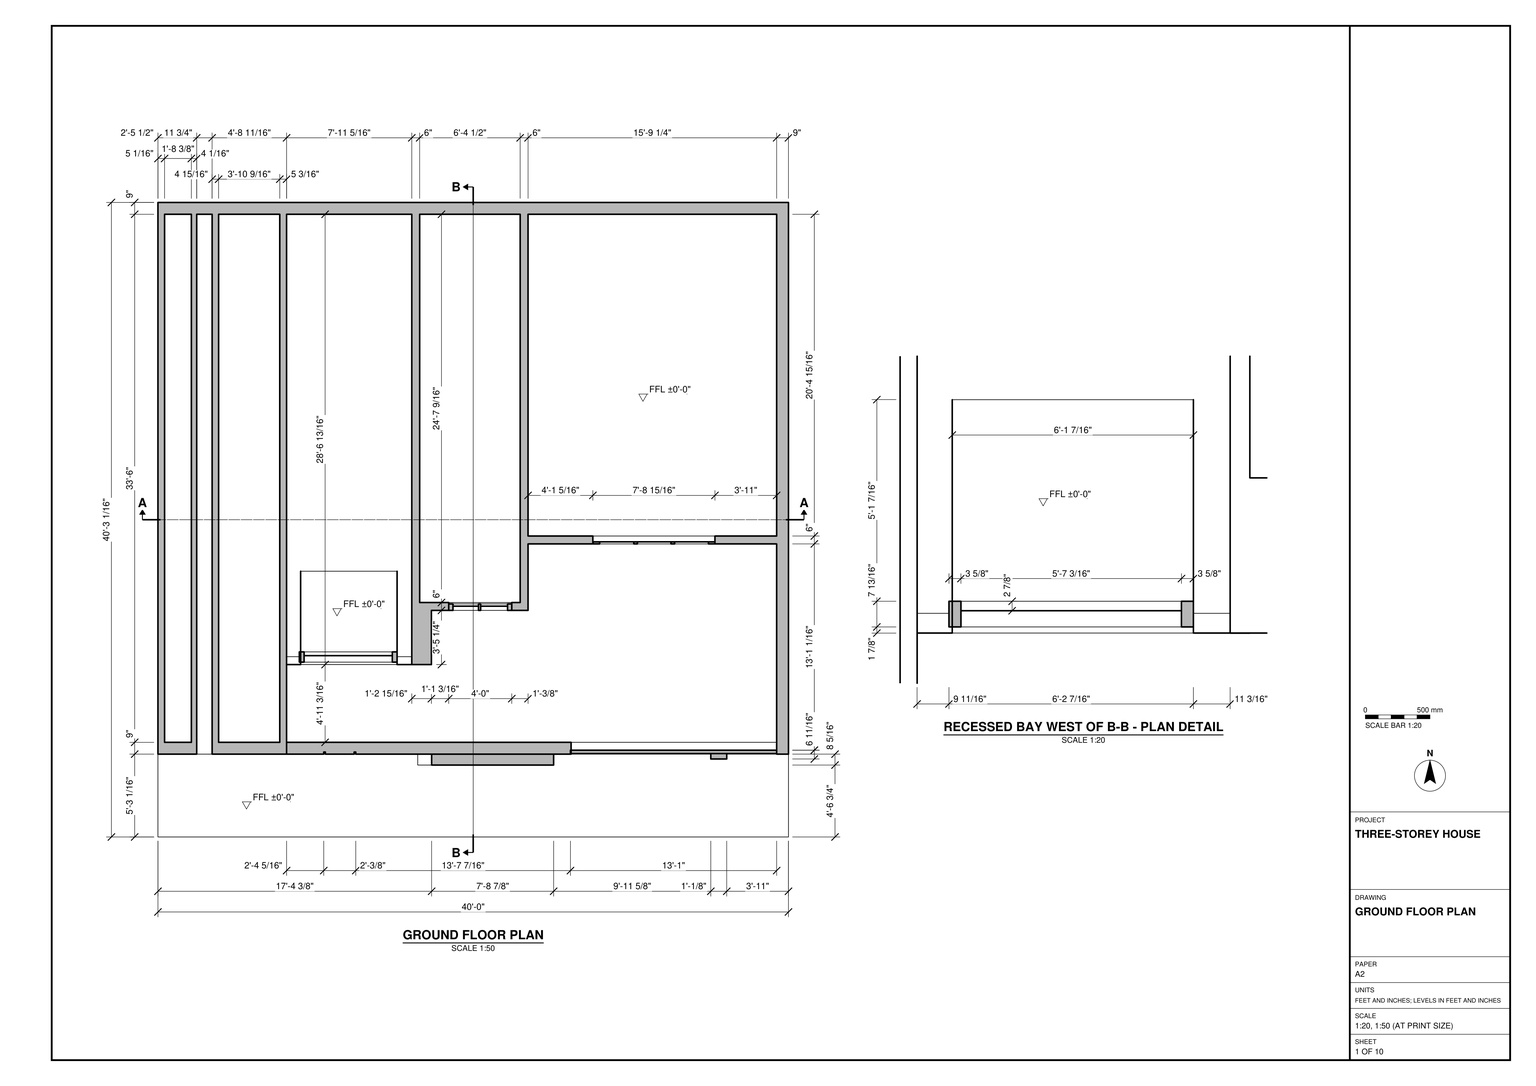
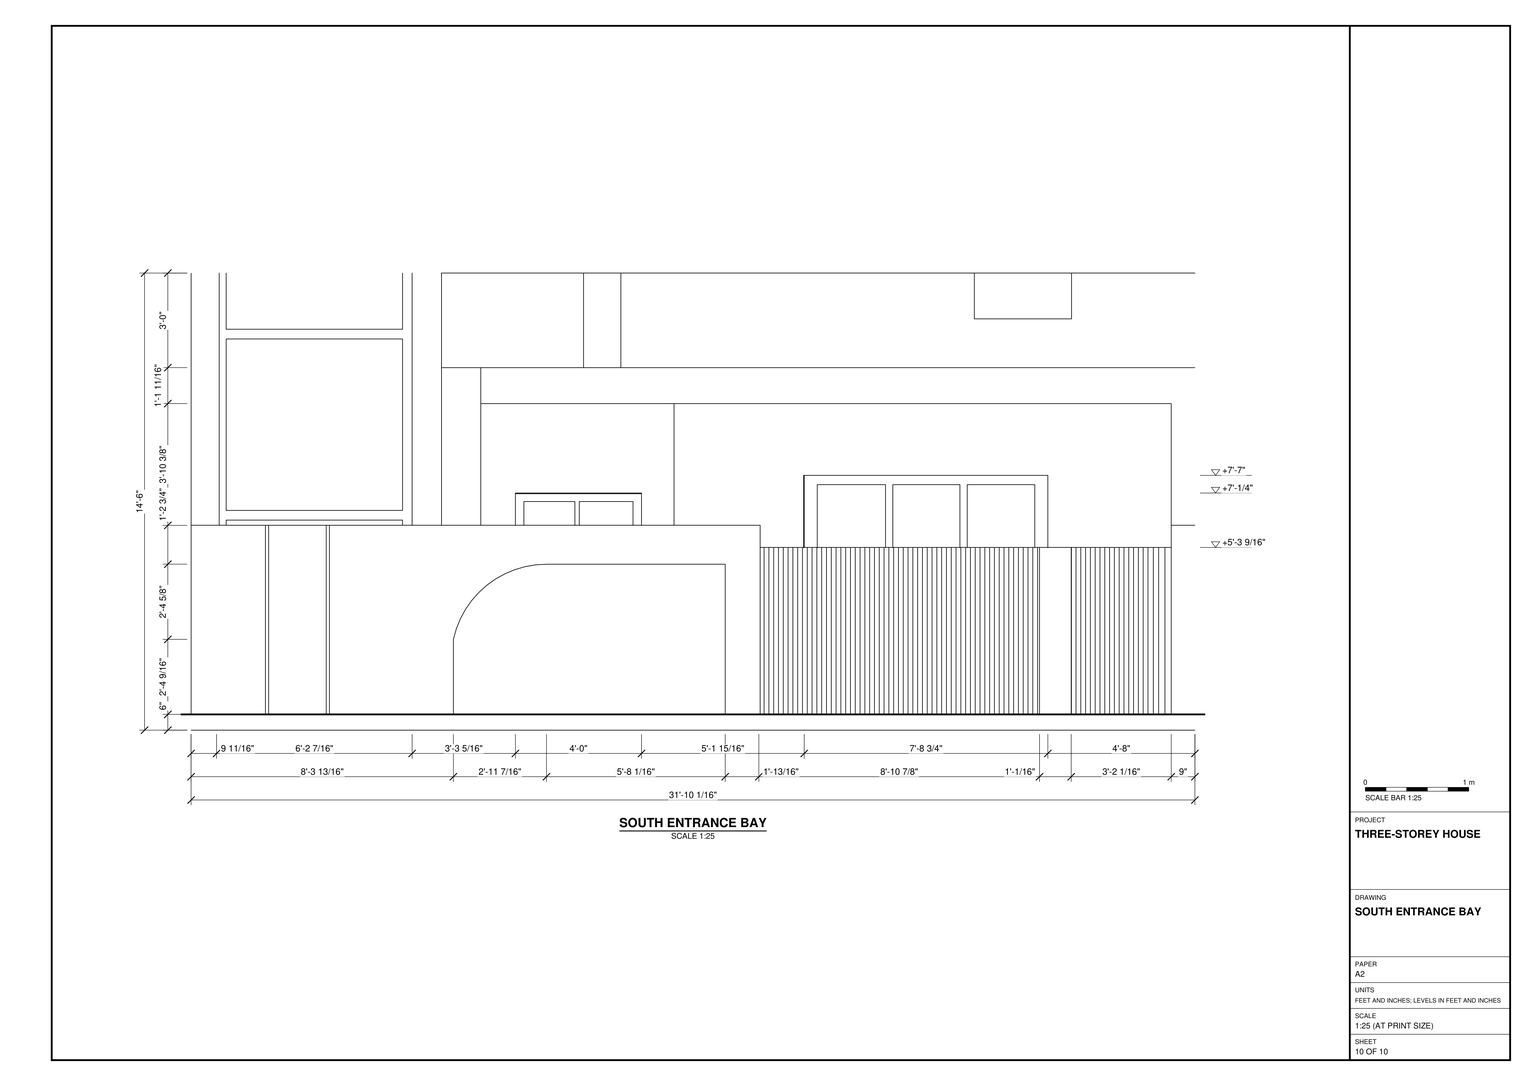
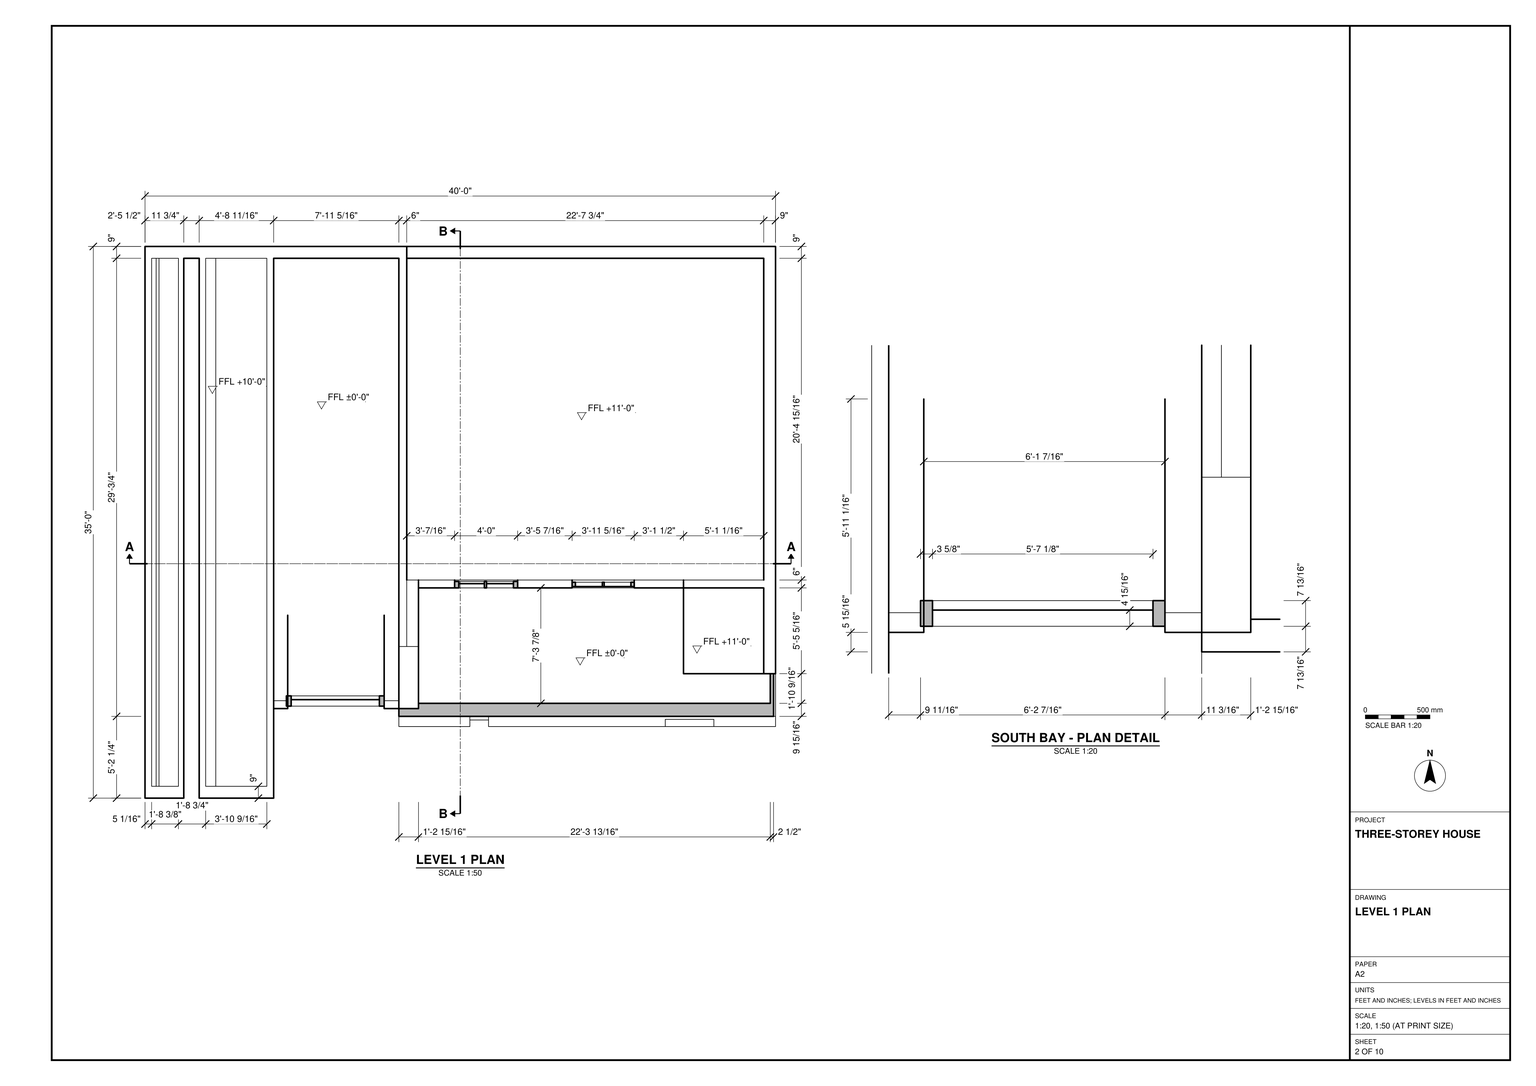
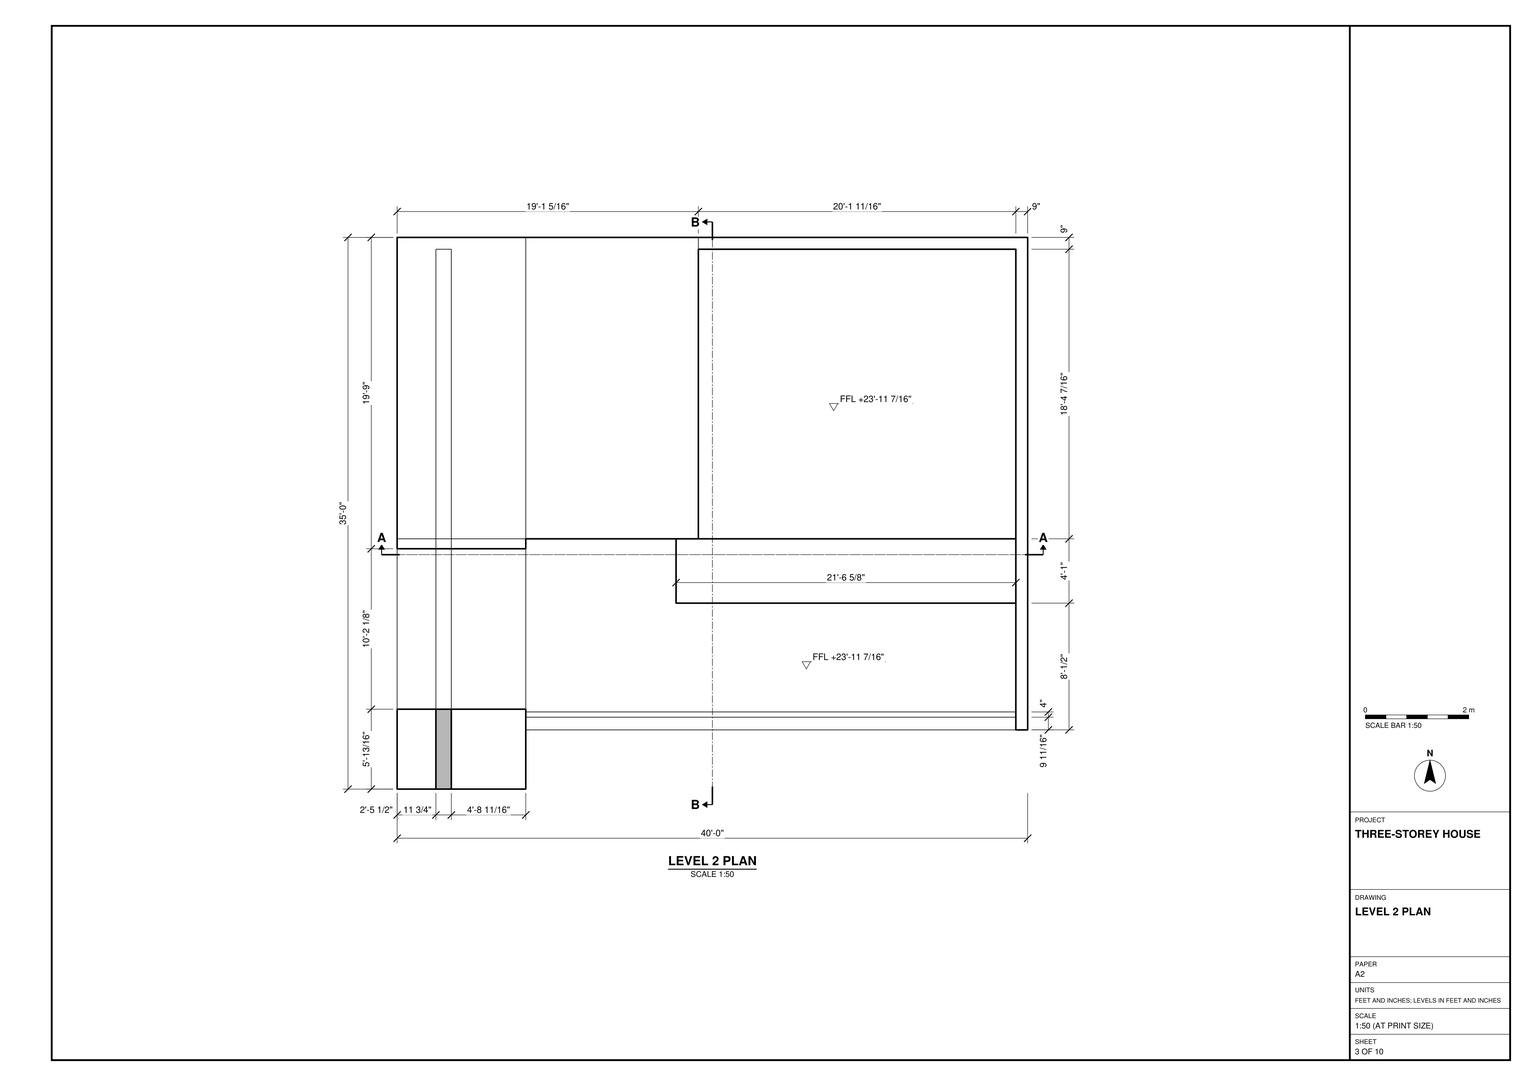
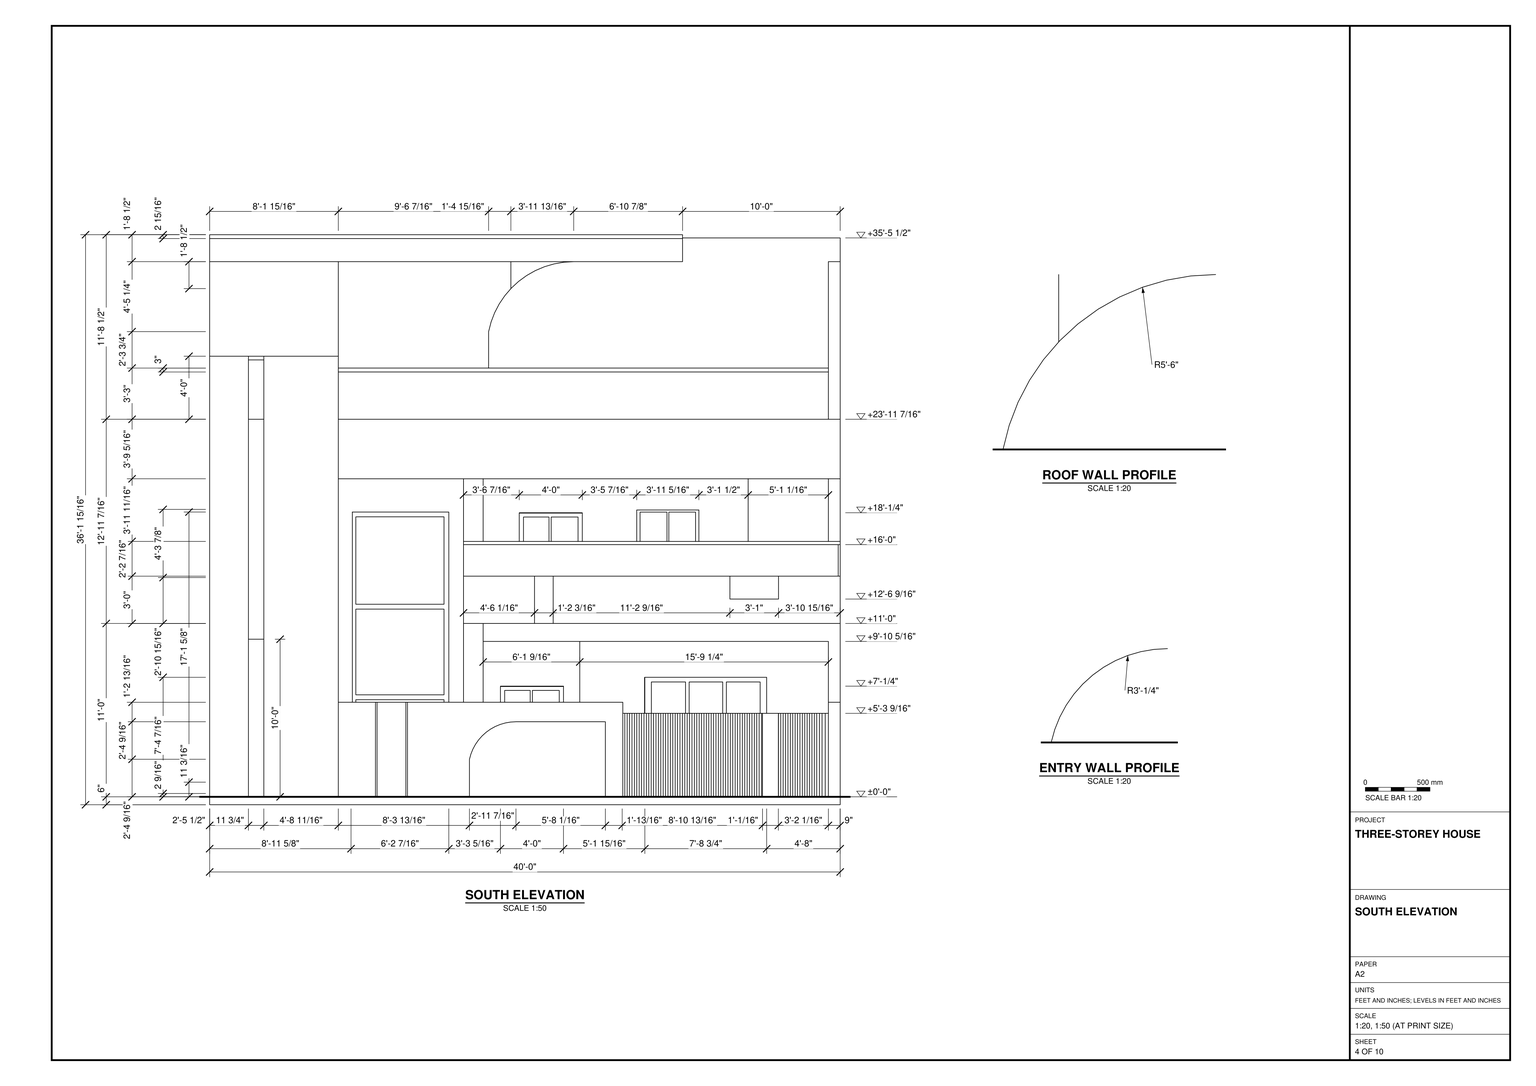
Build the three-storey house in SketchUp using task_files/diagram_01.pdf. Work in feet and inches. The overall model measures 40'-0" east to west, 40'-3 1/16" north to south and 36'-1 15/16" high. Set the finished floor levels at ±0'-0", +11'-0" and +23'-11 7/16".

Use the plans to lay out the long, narrow bays on the west and the wider spaces on the east. Give walls their drawn thicknesses, including 9" and 6" where marked. Form the recessed south bay with its opening set between the side returns. Use each storey's own slab outline rather than copying the ground floor upwards. Preserve the areas open to the floor below, and follow the sheets for the upper walls, openings, stairs and roof.

Use the enlarged south entrance drawing to position the framed openings behind the entrance screen. Match the curved corner profile in the solid portion and the two runs of closely spaced vertical members to its right. Include built-in joinery and main furniture where shown. Keep walls, slabs, roof elements and each furniture or joinery piece in separate groups or components, and use components for repeated parts. Any decor or loose items shown may use suitable library components. Save one SketchUp model as output_files/three_storey_house_with_a_screened_south_entrance.skp.

# SketchUp Ruby script. Lengths in inches.
U = 1.inch
M = Sketchup.active_model
def pt(a) = Geom::Point3d.new(a.map { |v| v * U })
def face(e, loops, mat)
  f = e.add_face(loops[0].map { |a| pt(a) })
  loops[1..].each { |l| e.add_face(l.map { |a| pt(a) }).erase! }
  f.material = f.back_material = mat if mat
  f
end
# faces: each face lists its corners as indices into pts; further lists are holes
def faces(e, pts, list, mat = nil) = list.each { |f| face(e, (f[0].is_a?(Array) ? f : [f]).map { |l| l.map { |i| pts[i] } }, mat) }
# xy, xz, yz: faces in a plane at the given z, y or x. An outline is a flat list of corners, or four numbers for a rectangle; further outlines are holes
def ring(l) = l.size == 4 ? [[l[0], l[1]], [l[2], l[1]], [l[2], l[3]], [l[0], l[3]]] : l.each_slice(2).to_a
def flat(e, list, mat, &to3) = list.each { |f| face(e, (f[0].is_a?(Array) ? f : [f]).map { |l| ring(l).map { |u, v| to3.(u, v) } }, mat) }
def xy(e, z, list, mat = nil) = flat(e, list, mat) { |x, y| [x, y, z] }
def xz(e, y, list, mat = nil) = flat(e, list, mat) { |x, z| [x, y, z] }
def yz(e, x, list, mat = nil) = flat(e, list, mat) { |y, z| [x, y, z] }
def lines(e, pts, list) = list.each { |a, b| e.add_line(pt(pts[a]), pt(pts[b])) }
# prism: a flat outline (further loops are holes) pulled along v
def prism(e, loops, v, mat = nil)
  f = face(e, loops, mat); d = Geom::Vector3d.new(v.map { |x| x * U })
  f.pushpull(f.normal.samedirection?(d) ? d.length : -d.length)
end
def box(e, o, s, mat = nil) = prism(e, [[o, [o[0] + s[0], o[1], o[2]], [o[0] + s[0], o[1] + s[1], o[2]], [o[0], o[1] + s[1], o[2]]]], [0, 0, s[2]], mat)
def at(x, y, z, deg = 0) = Geom::Transformation.translation(pt([x, y, z])) * Geom::Transformation.rotation(ORIGIN, Z_AXIS, deg.degrees)
def axes(o, x, y, z) = Geom::Transformation.new([*x, 0, *y, 0, *z, 0, *pt(o).to_a, 1])
def part(name) = M.definitions.add(name)
# library, detail: a bought-in or finely detailed component or shape, given as its bounding box
def library(name, o, s) = part(name).tap { |d| box(d.entities, o, s) }
def detail(e, o, s) = box(e.add_group.entities, o, s)
def put(e, d, t, mat = nil) = e.add_instance(d, t).tap { |i| i.material = mat if mat }
def group(e, t, mat = nil) = e.add_group.tap { |g| g.transformation = t; g.material = mat if mat }.entities
root = M.entities
M.materials.add("[Color B04]").color = [229, 179, 115]
M.materials.add("[Color B08]").color = [73, 25, 0]
M.materials.add("[Color C02]").color = [255, 204, 153]
M.materials.add("[Color C07]").color = [102, 54, 0]
M.materials.add("[Color M00]").color = [255, 255, 255]
M.materials.add("[Color M05]").color = [114, 114, 114]
M.materials.add("[Concrete Aggregate Smoke]").color = [154, 150, 148]
M.materials.add("[Concrete Form 4x8]").color = [167, 170, 168]
M.materials.add("[Field Rectangle Tile]").color = [196, 189, 179]
M.materials.add("[Field Square Tile]").color = [217, 201, 169]
M.materials.add("[Marble Carrara Gold Floor Tile]").color = [225, 223, 217]
M.materials.add("[Marble Carrara Gold Floor Tile]1").color = [225, 223, 217]
M.materials.add("[Sandstone]").color = [118, 81, 52]
M.materials.add("[Stone Brushed Khaki]").color = [226, 197, 133]
M.materials.add("[Stone Marble]").color = [143, 138, 136]
M.materials.add("[Translucent Glass Blue]").color = [223, 205, 74]
M.materials["[Translucent Glass Blue]"].alpha = 0.5
M.materials.add("[Translucent Glass Gray]").color = [128, 128, 128]
M.materials["[Translucent Glass Gray]"].alpha = 0.5
c1 = part("Group\#3")
xy(c1.entities,0,[[0,0,48,6.5]],"[Color C07]")
xy(c1.entities,3.23,[[22.64,0,24.3125,6.5]])
xy(c1.entities,3.23,[[3.23,0,22.64,4.25],[24.3125,0,44.77,4.25],[3.23,4.25,22.64,6.5],[24.3125,4.25,44.77,6.5]],"[Color C07]")
xy(c1.entities,80.77,[[3.23,0,22.64,4.25],[24.3125,0,44.77,4.25],[3.23,4.25,22.64,6.5],[24.3125,4.25,44.77,6.5]],"[Color C07]")
xy(c1.entities,84,[[0,0,48,6.5]],"[Color C07]")
xz(c1.entities,0,[[[0,0,48,84],[3.23,3.23,3.23,80.77,22.64,80.77,22.64,3.23,24.3125,3.23,24.3125,80.77,44.77,80.77,44.77,3.23]]],"[Color C07]")
xz(c1.entities,4.25,[[3.23,3.23,22.64,80.77],[24.3125,3.23,44.77,80.77]],"[Color C07]")
xz(c1.entities,6.5,[[[0,0,48,84],[3.23,3.23,44.77,3.23,44.77,80.77,24.3125,80.77,24.3125,3.23,22.64,3.23,22.64,80.77,3.23,80.77]]],"[Color C07]")
yz(c1.entities,0,[[0,0,6.5,84]],"[Color C07]")
yz(c1.entities,3.23,[[0,3.23,4.25,80.77],[4.25,3.23,6.5,80.77]],"[Color C07]")
yz(c1.entities,22.64,[[0,3.23,4.25,80.77],[4.25,3.23,6.5,80.77]],"[Color C07]")
yz(c1.entities,24.3125,[[0,3.23,4.25,80.77],[4.25,3.23,6.5,80.77]],"[Color C07]")
yz(c1.entities,44.77,[[0,3.23,4.25,80.77],[4.25,3.23,6.5,80.77]],"[Color C07]")
yz(c1.entities,48,[[0,0,6.5,84]],"[Color C07]")
xy(root,0,[[0,0,480,63.0625],[0,63.0625,480,483.0625]],"[Concrete Form 4x8]")
xy(root,6,[[[0,63.0625,0,483.0625,45.375,483.0625,45.375,474.0625,29.52,474.0625,29.52,63.0625],[5.0625,72.0625,25.4375,474.0625]],[29.52,63.0625,41.25,474.0625],[41.25,63.0625,41.25,474.0625,45.375,474.0625,45.375,483.0625,75.0625,483.0625,75.0625,474.0625,46.1875,474.0625,46.1875,72.0625,97.9375,72.0625,97.9375,63.0625],[97.9375,63.0625,97.9375,72.0625,314.52,72.0625,314.52,63.0625,150.59,63.0625,150.59,64.6875,149.37,64.6875,149.37,63.0625,127.44,63.0625,127.44,64.6875,126.22,64.6875,126.22,63.0625],[126.22,63.0625,127.44,64.6875],
  [149.37,63.0625,150.59,64.6875],[314.52,63.0625,471,72.0625],[471,63.0625,480,131.25],[5.0625,72.0625,25.4375,474.0625],[46.1875,72.0625,92.75,474.0625],
  [92.75,72.0625,97.9375,474.0625],[193.25,131.08,199.25,131.25],[[193.25,131.25,193.25,474.0625,75.0625,474.0625,75.0625,483.0625,480,483.0625,480,147.59,471,147.59,471,223.125,281.75,223.125,281.75,172.5,269.37,172.5,269.37,178.5,275.75,178.5,275.75,474.0625,199.25,474.0625,199.25,178.5,221.37,178.5,221.37,172.5,208.1875,172.5,208.1875,131.25],[281.75,229.125,471,474.0625]],[97.9375,131.25,193.25,137.25],[471,131.25,480,147.59],
  [97.9375,137.25,193.25,474.0625],[199.25,178.5,275.75,474.0625],[281.75,229.125,471,474.0625]])
xy(root,6,[[97.9375,72.0625,471,72.0625,471,223.125,281.75,223.125,281.75,172.5,269.37,172.5,269.37,178.5,221.37,178.5,221.37,172.5,208.1875,172.5,208.1875,131.25,199.25,131.25,199.25,131.08,193.25,131.08,193.25,131.25,97.9375,131.25]],"[Concrete Aggregate Smoke]")
xy(root,6,[[0,0,480,0,480,63.0625,301.23,63.0625,301.23,54.75,197.77,54.75,197.77,63.0625,0,63.0625]],"[Concrete Form 4x8]")
xy(root,6,[[197.77,54.75,301.23,63.0625]],"[Marble Carrara Gold Floor Tile]1")
xy(root,8.56,[[331.09,223.125,424.02,229.125]])
xy(root,17.18,[[108.62,131.25,182.06,202.3125]],"[Color M00]")
xy(root,63.17,[[233.21,54.75,301.23,63.0625]],"[Marble Carrara Gold Floor Tile]1")
xy(root,78,[[97.9375,63.0625,126.22,63.0625,126.22,64.6875,127.44,64.6875,127.44,63.0625,149.37,63.0625,149.37,64.6875,150.59,64.6875,150.59,63.0625,314.52,63.0625,314.52,72.0625,97.9375,72.0625]],"[Field Square Tile]")
xy(root,78,[[471,63.0625,480,131.25]],"[Stone Marble]")
xy(root,90,[[221.37,172.5,269.37,178.5]])
xy(root,97,[[331.09,223.125,424.02,229.125]])
xy(root,119.125,[[46.1875,72.0625,92.75,474.0625]])
xy(root,119.625,[[5.0625,72.0625,25.4375,474.0625]])
xy(root,124.3125,[[208.1875,131.25,208.1875,172.5,281.75,172.5,281.75,223.125,471,223.125,471,131.25]],"[Color M00]")
xy(root,126,[[5.0625,72.0625,8.47,474.0625],[8.47,72.0625,10.66,474.0625],[10.66,72.0625,25.4375,474.0625],[46.1875,72.0625,53.875,474.0625],[53.875,72.0625,92.75,474.0625]])
xy(root,133.8125,[[199.25,229.125,275.75,474.0625]])
xy(root,135.5,[[281.75,229.125,471,474.0625]])
xy(root,138,[[471,157.8125,471,223.125,409.9375,223.125,409.9375,229.125,471,229.125,471,474.0625,199.25,474.0625,199.25,483.0625,480,483.0625,480,157.8125],[409.9375,157.8125,471,223.125],[199.25,178.5,208.1875,229.125],[208.1875,223.125,235.68,229.125],[283.68,223.125,409.9375,229.125],
  [199.25,229.125,471,474.0625]])
xy(root,138,[[193.25,117.5625,193.25,131.25,480,131.25,480,117.5625,261.51,117.5625,261.51,122.5625,247.3,122.5625,247.3,117.5625],[208.1875,131.25,208.1875,135.25,476,135.25,476,157.8125,480,157.8125,480,131.25],[208.1875,135.25,208.1875,223.125,235.68,223.125,235.68,229.125,283.68,229.125,283.68,223.125,409.9375,223.125,409.9375,157.8125,476,157.8125,476,135.25]],"[Color M00]")
xy(root,156.5625,[[396.06,117.5625,433.06,123.0625]],"[Stone Brushed Khaki]")
xy(root,172.95,[[325.125,223.125,372.4375,229.125]])
xy(root,174,[[193.25,125.3125,193.25,131.25,208.1875,131.25,208.1875,135.25,476,135.25,476,157.8125,478.5,157.8125,478.5,125.3125]],"[Color M00]")
xy(root,174,[[247.3,122.5625,261.51,125.3125]],"[Stone Brushed Khaki]")
xy(root,174,[[193.25,117.5625,247.3,125.3125],[261.51,117.5625,261.51,125.3125,480,125.3125,480,117.5625,433.06,117.5625,433.06,123.0625,396.06,123.0625,396.06,117.5625],[478.5,125.3125,480,157.8125]],"[Translucent Glass Gray]")
xy(root,198,[[193.25,125.3125,193.25,131.25,208.1875,131.25,208.1875,135.25,476,135.25,476,157.8125,478.5,157.8125,478.5,125.3125]],"[Color C02]")
xy(root,198,[[193.25,122.1875,480,125.3125],[478.5,125.3125,480,157.8125]],"[Translucent Glass Gray]")
xy(root,200.4375,[[193.25,122.1875,480,122.1875,480,157.8125,476,157.8125,476,135.25,208.1875,135.25,208.1875,131.25,193.25,131.25]],"[Color C02]")
xy(root,222,[[235.68,223.125,283.68,229.125]])
xy(root,222.8,[[108.62,131.25,182.06,202.3125]],"[Color M00]")
xy(root,224.38,[[325.125,223.125,372.4375,229.125]])
xy(root,248.125,[[97.9375,108.125,480,131.25]])
xy(root,257.4375,[[193.25,131.25,193.25,474.0625,97.9375,474.0625,97.9375,483.0625,199.25,483.0625,199.25,229.125,208.1875,229.125,208.1875,131.25],[97.9375,131.25,193.25,137.25],[208.1875,131.25,409.9375,223.125],[409.9375,131.25,480,157.8125],[471,157.8125,471,223.125,409.9375,223.125,409.9375,229.125,471,229.125,471,474.0625,199.25,474.0625,199.25,483.0625,480,483.0625,480,157.8125],
  [409.9375,157.8125,471,223.125],[208.1875,223.125,409.9375,229.125]])
xy(root,289.4375,[[199.25,229.125,471,474.0625]])
xy(root,289.625,[[97.9375,137.25,193.25,474.0625]])
xy(root,293.4375,[[97.9375,108.125,471,117.8125],[471,108.125,471,474.0625,229.3125,474.0625,229.3125,483.0625,480,483.0625,480,108.125],[97.9375,117.8125,471,121.8125],[97.9375,121.8125,471,121.8125,471,204.63,212.35,204.63,212.35,253.6,97.9375,253.6],[0,123.89,29.52,246.04],
  [41.25,123.89,97.9375,246.04],[212.35,204.63,471,253.6],[29.52,246.04,41.25,253.6],[41.25,246.04,97.9375,253.6],[97.9375,253.6,229.3125,483.0625],
  [229.3125,253.6,471,474.0625]])
xy(root,293.4375,[[29.52,123.89,41.25,246.04],[29.52,253.6,41.25,474.0625]],"[Color M00]")
xy(root,329.4375,[[97.9375,117.8125,471,121.8125]],"[Color C02]")
xy(root,332.4375,[[97.9375,117.8125,471,121.8125]],"[Color C02]")
xy(root,338.625,[[29.52,63.0625,41.25,123.89]],"[Color B04]")
xy(root,341.4375,[[0,63.0625,29.52,123.89],[29.52,63.0625,41.25,123.89],[41.25,63.0625,97.9375,123.89]],"[Color B04]")
xy(root,413.4375,[[277.12,204.63,360,253.6],[471,204.63,480,253.6],[0,246.04,97.9375,253.6],[0,253.6,0,483.0625,360,483.0625,360,474.0625,229.3125,474.0625,229.3125,253.6],[471,253.6,480,253.6,480,483.0625,360,483.0625,360,474.0625,471,474.0625]])
xy(root,413.4375,[[0,185.92,0,246.04,97.9375,246.04,97.9375,253.6,229.3125,253.6,229.3125,474.0625,360,474.0625,360,253.6,277.12,253.6,277.12,204.63,360,204.63,360,185.92]],"[Color M05]")
xy(root,413.4375,[[471,108.125,480,204.63]],"[Stone Marble]")
xy(root,431,[[0,178.35,360,185.92],[0,185.92,360,483.0625]],"[Color M05]")
xy(root,431.5,[[360,204.63,480,253.6]],"[Color B04]")
xy(root,433.9375,[[0,178.35,360,483.0625]],"[Color M05]")
xz(root,0,[[0,0,480,6]],"[Concrete Form 4x8]")
xz(root,54.75,[[197.77,6,301.23,6,301.23,63.17,233.21,63.17,229.11,62.94,225.07,62.25,221.14,61.1,217.35,59.52,213.77,57.52,210.44,55.13,207.4,52.38,204.69,49.31,202.34,45.95,200.39,42.34,198.86,38.54,197.77,34.59]],"[Marble Carrara Gold Floor Tile]1")
xz(root,63.0625,[[0,0,480,6]])
xz(root,63.0625,[[0,6,29.52,341.4375],[41.25,6,97.9375,341.4375],[29.52,338.625,41.25,341.4375]],"[Color B04]")
xz(root,63.0625,[[97.9375,6,126.22,78],[127.44,6,149.37,78],[150.59,6,197.77,6,197.77,34.59,198.86,38.54,200.39,42.34,202.34,45.95,204.69,49.31,207.4,52.38,210.44,55.13,213.77,57.52,217.35,59.52,221.14,61.1,225.07,62.25,229.11,62.94,233.21,63.17,301.23,63.17,301.23,6,314.52,6,314.52,78,150.59,78]],"[Field Square Tile]")
xz(root,63.0625,[[197.77,6,197.77,34.59,198.86,38.54,200.39,42.34,202.34,45.95,204.69,49.31,207.4,52.38,210.44,55.13,213.77,57.52,217.35,59.52,221.14,61.1,225.07,62.25,229.11,62.94,233.21,63.17,301.23,63.17,301.23,6]],"[Marble Carrara Gold Floor Tile]1")
xz(root,63.0625,[[471,6,480,78]],"[Stone Marble]")
xz(root,64.6875,[[126.22,6,127.44,78],[149.37,6,150.59,78]],"[Field Square Tile]")
xz(root,72.0625,[[5.0625,6,25.4375,119.625],[46.1875,6,92.75,119.125],[97.9375,6,117.6875,78],[117.6875,6,123.6875,78],[123.6875,6,314.52,78],
  [46.1875,119.125,92.75,126],[5.0625,119.625,25.4375,126]])
xz(root,108.125,[[97.9375,248.125,480,293.4375]])
xz(root,108.125,[[471,293.4375,480,413.4375]],"[Stone Marble]")
xz(root,117.5625,[[193.25,138,247.3,174],[261.51,138,480,138,480,174,433.06,174,433.06,156.5625,396.06,156.5625,396.06,174,261.51,174]],"[Color M00]")
xz(root,117.8125,[[97.9375,329.4375,471,332.4375]],"[Color C02]")
xz(root,117.8125,[[97.9375,293.4375,471,329.4375]],"[Translucent Glass Gray]")
xz(root,121.8125,[[97.9375,329.4375,471,332.4375]],"[Color C02]")
xz(root,121.8125,[[97.9375,293.4375,471,329.4375]],"[Translucent Glass Gray]")
xz(root,122.1875,[[193.25,198,480,200.4375]],"[Color C02]")
xz(root,122.5625,[[247.3,138,261.51,174]],"[Stone Brushed Khaki]")
xz(root,123.0625,[[396.06,156.5625,433.06,174]],"[Stone Brushed Khaki]")
xz(root,123.89,[[29.52,338.625,41.25,341.4375]])
xz(root,123.89,[[0,293.4375,29.52,341.4375],[29.52,293.4375,41.25,338.625],[41.25,293.4375,97.9375,341.4375]],"[Color B04]")
xz(root,125.3125,[[193.25,174,478.5,198]],"[Translucent Glass Gray]")
xz(root,131.08,[[193.25,2.25,199.25,6]])
xz(root,131.25,[[193.25,138,208.1875,174],[97.9375,248.125,193.25,257.4375],[193.25,248.125,208.1875,257.4375],[208.1875,248.125,409.9375,257.4375],[409.9375,248.125,480,257.4375]])
xz(root,131.25,[[193.25,198,208.1875,200.4375]],"[Color C02]")
xz(root,131.25,[[[97.9375,6,193.25,248.125],[108.62,17.18,182.06,222.8]],[193.25,6,208.1875,138],[471,78,480,78,480,138,208.1875,138,208.1875,124.3125,471,124.3125],[193.25,174,208.1875,198],[193.25,200.4375,208.1875,248.125]],"[Stone Marble]")
xz(root,135.25,[[208.1875,198,476,200.4375]],"[Color C02]")
xz(root,135.25,[[208.1875,138,476,174]],"[Color M00]")
xz(root,135.25,[[208.1875,174,476,198]],"[Translucent Glass Gray]")
xz(root,137.25,[[97.9375,257.4375,193.25,289.625]])
xz(root,147.59,[[471,2.25,480,6]])
xz(root,157.8125,[[476,198,480,200.4375]],"[Color C02]")
xz(root,157.8125,[[476,138,480,174],[476,174,478.5,198]],"[Color M00]")
xz(root,157.8125,[[409.9375,138,471,257.4375],[471,138,476,138,476,200.4375,480,200.4375,480,257.4375,471,257.4375]],"[Marble Carrara Gold Floor Tile]")
xz(root,157.8125,[[478.5,174,480,198]],"[Translucent Glass Gray]")
xz(root,172.5,[[208.1875,6,221.37,6,221.37,90,269.37,90,269.37,6,281.75,6,281.75,124.3125,208.1875,124.3125]],"[Stone Brushed Khaki]")
xz(root,178.35,[[0,431,360,433.9375]],"[Color M05]")
xz(root,178.5,[[199.25,6,199.25,126,275.75,126,275.75,6,269.37,6,269.37,90,221.37,90,221.37,6]])
xz(root,185.92,[[0,413.4375,360,431]],"[Color M05]")
xz(root,204.63,[[212.35,293.4375,471,293.4375,471,413.4375,480,413.4375,480,431.5,360,431.5,360,413.4375,277.12,413.4375,269.5625,413,262.11,411.71,254.85,409.57,247.88,406.61,241.3,402.87,235.1875,398.41,229.625,393.27,224.69,387.53,220.44,381.27,216.94,374.56,214.23,367.49,212.35,360.16]],"[Color B04]")
xz(root,223.125,[[409.9375,138,471,257.4375]])
xz(root,223.125,[[[281.75,6,471,124.3125],[331.09,8.56,424.02,97]],[[208.1875,138,235.68,138,235.68,222,283.68,222,283.68,138,409.9375,138,409.9375,257.4375,208.1875,257.4375],[325.125,172.95,372.4375,224.38]]],"[Stone Brushed Khaki]")
xz(root,229.125,[[[281.75,6,471,126],[331.09,8.56,424.02,97]],[275.75,126,281.75,138],[281.75,126,471,135.5],[199.25,133.8125,275.75,138],[281.75,135.5,471,138],
  [199.25,257.4375,208.1875,289.4375],[208.1875,257.4375,275.75,289.4375],[275.75,257.4375,281.75,289.4375],[281.75,257.4375,471,289.4375]])
xz(root,246.04,[[0,293.4375,97.9375,413.4375]],"[Stone Brushed Khaki]")
xz(root,253.6,[[212.35,293.4375,229.3125,293.4375,229.3125,392.91,224.69,387.53,220.44,381.27,216.94,374.56,214.23,367.49,212.35,360.16]])
xz(root,253.6,[[229.3125,293.4375,229.3125,392.91,229.625,393.27,235.1875,398.41,241.3,402.87,247.88,406.61,254.85,409.57,262.11,411.71,269.5625,413,277.12,413.4375,471,413.4375,471,293.4375],[360,413.4375,480,431.5]],"[Color B04]")
xz(root,253.6,[[97.9375,293.4375,212.35,293.4375,212.35,360.16,214.23,367.49,216.94,374.56,220.44,381.27,224.69,387.53,229.3125,392.91,229.3125,413.4375,97.9375,413.4375]],"[Field Rectangle Tile]")
xz(root,474.0625,[[123.6875,2.25,193.25,6],[199.25,2.25,275.75,6],[281.75,2.25,471,6],[5.0625,6,25.4375,119.625],[29.52,6,41.25,126],
  [46.1875,6,92.75,119.125],[97.9375,6,193.25,257.4375],[199.25,6,275.75,126],[281.75,6,471,126],[275.75,90,281.75,126],
  [46.1875,119.125,53.875,126],[53.875,119.125,92.75,126],[5.0625,119.625,8.47,126],[8.47,119.625,10.66,126],[10.66,119.625,25.4375,126],
  [29.52,126,41.25,293.4375],[199.25,126,275.75,133.8125],[275.75,126,281.75,138],[281.75,126,471,135.5],[199.25,133.8125,275.75,138],
  [281.75,135.5,291.9375,138],[291.9375,135.5,471,138],[199.25,138,471,257.4375],[97.9375,257.4375,193.25,289.625],[199.25,257.4375,471,289.4375],
  [240.25,289.4375,471,293.4375],[229.3125,293.4375,471,413.4375]])
xz(root,483.0625,[[0,6,9,126],[9,6,45.375,126],[45.375,6,75.0625,126],[75.0625,6,480,126],[0,126,9,413.4375],
  [9,126,45.375,413.4375],[45.375,126,75.0625,413.4375],[75.0625,126,75.0625,413.4375,97.9375,413.4375,97.9375,257.4375,199.25,257.4375,199.25,126],[199.25,126,480,138],[199.25,138,480,257.4375],
  [97.9375,257.4375,199.25,293.4375],[199.25,257.4375,480,293.4375],[97.9375,293.4375,199.25,413.4375],[199.25,293.4375,480,413.4375]],"[Color B04]")
xz(root,483.0625,[[0,413.4375,360,431],[0,431,360,433.9375]],"[Color M05]")
xz(root,483.0625,[[0,0,480,6]],"[Concrete Form 4x8]")
yz(root,0,[[63.0625,6,63.0625,341.4375,123.89,341.4375,123.89,293.4375,246.04,293.4375,246.04,413.4375,483.0625,413.4375,483.0625,6]],"[Color B04]")
yz(root,0,[[185.92,413.4375,483.0625,431],[178.35,431,483.0625,433.9375]],"[Color M05]")
yz(root,0,[[0,0,63.0625,6],[63.0625,0,483.0625,6]],"[Concrete Form 4x8]")
yz(root,5.0625,[[72.0625,6,474.0625,119.625],[72.0625,119.625,474.0625,126]])
yz(root,25.4375,[[72.0625,6,474.0625,119.625],[72.0625,119.625,474.0625,126]])
yz(root,29.52,[[63.0625,338.625,123.89,341.4375]])
yz(root,29.52,[[63.0625,6,474.0625,6,474.0625,293.4375,123.89,293.4375,123.89,338.625,63.0625,338.625]],"[Color B04]")
yz(root,41.25,[[63.0625,338.625,123.89,341.4375]])
yz(root,41.25,[[63.0625,6,63.0625,338.625,123.89,338.625,123.89,293.4375,474.0625,293.4375,474.0625,6]],"[Color B04]")
yz(root,46.1875,[[72.0625,6,474.0625,119.125],[72.0625,119.125,474.0625,126]])
yz(root,92.75,[[72.0625,6,474.0625,119.125],[72.0625,119.125,474.0625,126]])
yz(root,97.9375,[[63.0625,6,72.0625,78],[131.25,6,137.25,126],[137.25,6,474.0625,289.625],[131.25,126,137.25,257.4375],[108.125,248.125,131.25,248.125,131.25,257.4375,137.25,257.4375,137.25,293.4375,108.125,293.4375],
  [474.0625,257.4375,483.0625,293.4375],[137.25,289.625,474.0625,293.4375],[117.8125,293.4375,121.8125,329.4375]])
yz(root,97.9375,[[72.0625,6,131.25,6,131.25,248.125,108.125,248.125,108.125,293.4375,117.8125,293.4375,117.8125,332.4375,121.8125,332.4375,121.8125,293.4375,123.89,293.4375,123.89,341.4375,63.0625,341.4375,63.0625,78,72.0625,78]],"[Color B04]")
yz(root,97.9375,[[117.8125,329.4375,121.8125,332.4375]],"[Color C02]")
yz(root,97.9375,[[246.04,293.4375,253.6,413.4375]],"[Stone Brushed Khaki]")
yz(root,108.62,[[131.25,17.18,202.3125,222.8]],"[Color M00]")
yz(root,126.22,[[63.0625,6,64.6875,78]])
yz(root,127.44,[[63.0625,6,64.6875,78]])
yz(root,149.37,[[63.0625,6,64.6875,78]])
yz(root,150.59,[[63.0625,6,64.6875,78]])
yz(root,182.06,[[131.25,17.18,202.3125,222.8]],"[Color M00]")
yz(root,193.25,[[131.25,6,137.25,126],[137.25,6,474.0625,257.4375],[131.25,126,137.25,138],[131.25,138,137.25,257.4375],[137.25,257.4375,474.0625,289.625]])
yz(root,193.25,[[122.1875,198,131.25,200.4375]],"[Color C02]")
yz(root,193.25,[[117.5625,138,131.25,174]],"[Color M00]")
yz(root,193.25,[[125.3125,174,131.25,198]],"[Translucent Glass Gray]")
yz(root,197.77,[[54.75,6,63.0625,34.59]],"[Marble Carrara Gold Floor Tile]1")
yz(root,199.25,[[178.5,6,474.0625,126],[178.5,126,474.0625,126,474.0625,133.8125,229.125,133.8125,229.125,138,178.5,138],[474.0625,126,483.0625,138],[229.125,133.8125,474.0625,138],[229.125,138,474.0625,257.4375],
  [474.0625,138,483.0625,257.4375],[229.125,257.4375,474.0625,289.4375]])
yz(root,208.1875,[[223.125,138,229.125,257.4375]])
yz(root,208.1875,[[131.25,198,135.25,200.4375]],"[Color C02]")
yz(root,208.1875,[[131.25,138,135.25,174],[131.25,174,135.25,198]],"[Color M00]")
yz(root,208.1875,[[131.25,6,172.5,124.3125],[135.25,138,223.125,138,223.125,257.4375,131.25,257.4375,131.25,200.4375,135.25,200.4375]],"[Stone Marble]")
yz(root,212.35,[[204.63,293.4375,253.6,360.16]],"[Color B04]")
yz(root,221.37,[[172.5,6,178.5,90]])
yz(root,229.3125,[[253.6,293.4375,474.0625,413.4375]])
yz(root,235.68,[[223.125,138,229.125,222]])
yz(root,247.3,[[117.5625,138,122.5625,174]],"[Stone Brushed Khaki]")
yz(root,261.51,[[117.5625,138,122.5625,174]],"[Stone Brushed Khaki]")
yz(root,269.37,[[172.5,6,178.5,90]])
yz(root,275.75,[[178.5,6,178.5,126,393.3125,126,393.3125,90,474.0625,90,474.0625,6],[393.3125,90,402.4375,126],[402.4375,90,474.0625,126],[229.125,126,393.3125,133.8125],[393.3125,126,402.4375,133.8125],
  [402.4375,126,474.0625,133.8125]])
yz(root,281.75,[[229.125,6,474.0625,135.5]])
yz(root,281.75,[[172.5,6,223.125,124.3125]],"[Stone Brushed Khaki]")
yz(root,283.68,[[223.125,138,229.125,222]])
yz(root,301.23,[[54.75,6,63.0625,63.17]],"[Marble Carrara Gold Floor Tile]1")
yz(root,314.52,[[63.0625,6,72.0625,78]])
yz(root,325.125,[[223.125,172.95,229.125,224.38]])
yz(root,331.09,[[223.125,8.56,229.125,97]])
yz(root,360,[[204.63,413.4375,253.6,431],[204.63,431,253.6,431.5]])
yz(root,360,[[185.92,413.4375,204.63,431],[253.6,413.4375,483.0625,431],[178.35,431,204.63,433.9375],[253.6,431,483.0625,433.9375],[204.63,431.5,253.6,433.9375]],"[Color M05]")
yz(root,372.4375,[[223.125,172.95,229.125,224.38]])
yz(root,396.06,[[117.5625,156.5625,123.0625,174]],"[Stone Brushed Khaki]")
yz(root,409.9375,[[223.125,138,229.125,257.4375]])
yz(root,409.9375,[[157.8125,138,223.125,257.4375]],"[Marble Carrara Gold Floor Tile]")
yz(root,424.02,[[223.125,8.56,229.125,97]])
yz(root,433.06,[[117.5625,156.5625,123.0625,174]],"[Stone Brushed Khaki]")
yz(root,471,[[147.59,2.25,223.125,6],[229.125,2.25,474.0625,6],[229.125,6,474.0625,126],[229.125,126,474.0625,135.5],[229.125,135.5,474.0625,138],
  [157.8125,138,223.125,257.4375],[229.125,138,474.0625,257.4375],[229.125,257.4375,474.0625,289.4375],[117.8125,293.4375,121.8125,329.4375],[204.63,293.4375,253.6,413.4375],
  [253.6,293.4375,474.0625,413.4375]])
yz(root,471,[[117.8125,329.4375,121.8125,332.4375]],"[Color C02]")
yz(root,471,[[63.0625,6,63.0625,78,131.25,78,131.25,124.3125,223.125,124.3125,223.125,6],[108.125,293.4375,108.125,413.4375,204.63,413.4375,204.63,293.4375,121.8125,293.4375,121.8125,332.4375,117.8125,332.4375,117.8125,293.4375]],"[Stone Marble]")
yz(root,476,[[135.25,198,157.8125,200.4375]],"[Color C02]")
yz(root,476,[[135.25,138,157.8125,174]],"[Color M00]")
yz(root,476,[[135.25,174,157.8125,198]],"[Translucent Glass Gray]")
yz(root,478.5,[[125.3125,174,157.8125,198]],"[Translucent Glass Gray]")
yz(root,480,[[108.125,248.125,131.25,248.125,131.25,257.4375,157.8125,257.4375,157.8125,293.4375,108.125,293.4375]])
yz(root,480,[[131.25,6,483.0625,126],[131.25,126,483.0625,138],[157.8125,138,483.0625,257.4375],[157.8125,257.4375,483.0625,293.4375],[157.8125,293.4375,483.0625,413.4375],
  [204.63,413.4375,253.6,431.5]],"[Color B04]")
yz(root,480,[[122.1875,198,157.8125,200.4375]],"[Color C02]")
yz(root,480,[[117.5625,138,157.8125,174]],"[Color M00]")
yz(root,480,[[0,0,63.0625,6],[63.0625,0,147.59,6],[147.59,0,483.0625,6]],"[Concrete Form 4x8]")
yz(root,480,[[63.0625,6,131.25,78],[108.125,293.4375,157.8125,413.4375]],"[Stone Marble]")
p = [[198.86,63.0625,38.54],[197.77,63.0625,34.59],[197.77,54.75,34.59],[198.86,54.75,38.54],[200.39,63.0625,42.34],[200.39,54.75,42.34],
  [202.34,63.0625,45.95],[202.34,54.75,45.95],[204.69,63.0625,49.31],[204.69,54.75,49.31],[207.4,63.0625,52.38],[207.4,54.75,52.38],
  [210.44,63.0625,55.13],[210.44,54.75,55.13],[213.77,63.0625,57.52],[213.77,54.75,57.52],[217.35,63.0625,59.52],[217.35,54.75,59.52],
  [221.14,63.0625,61.1],[221.14,54.75,61.1],[225.07,63.0625,62.25],[225.07,54.75,62.25],[229.11,63.0625,62.94],[229.11,54.75,62.94],
  [233.21,63.0625,63.17],[233.21,54.75,63.17],[212.35,204.63,360.16],[214.23,204.63,367.49],[214.23,253.6,367.49],[212.35,253.6,360.16],
  [216.94,204.63,374.56],[216.94,253.6,374.56],[220.44,204.63,381.27],[220.44,253.6,381.27],[224.69,204.63,387.53],[224.69,253.6,387.53],
  [229.625,204.63,393.27],[229.625,253.6,393.27],[229.3125,253.6,392.91],[235.1875,204.63,398.41],[235.1875,253.6,398.41],[241.3,204.63,402.87],
  [241.3,253.6,402.87],[247.88,204.63,406.61],[247.88,253.6,406.61],[254.85,204.63,409.57],[254.85,253.6,409.57],[262.11,204.63,411.71],
  [262.11,253.6,411.71],[269.5625,204.63,413],[269.5625,253.6,413],[277.12,204.63,413.4375],[277.12,253.6,413.4375],[9,474.0625,6],
  [9,474.0625,2.25],[117.6875,474.0625,6],[117.6875,474.0625,2.25],[117.6875,72.0625,6],[117.6875,72.0625,2.25],[9,72.0625,6],
  [9,72.0625,2.25],[123.6875,72.0625,6],[123.6875,72.0625,2.25],[199.25,172.5,6],[199.25,172.5,2.25],[9,483.0625,2.25],
  [123.6875,63.0625,2.25],[123.6875,474.0625,2.25],[117.6875,474.0625,0],[117.6875,72.0625,0],[123.6875,72.0625,0],[123.6875,474.0625,0],
  [193.25,474.0625,2.25],[193.25,474.0625,0],[199.25,131.08,2.25],[199.25,131.08,0],[471,223.125,2.25],[471,223.125,0],
  [471,147.59,2.25],[471,147.59,0],[199.25,474.0625,2.25],[199.25,474.0625,0],[275.75,474.0625,2.25],[275.75,474.0625,0],
  [281.75,474.0625,2.25],[281.75,474.0625,0],[471,474.0625,2.25],[471,474.0625,0],[45.375,474.0625,6],[45.375,474.0625,126],
  [29.52,474.0625,6],[25.4375,474.0625,6],[199.25,178.5,126],[193.25,178.5,126],[193.25,137.25,126],[199.25,178.5,138],
  [193.25,178.5,138],[275.75,178.5,126],[275.75,178.5,138],[199.25,178.5,246],[182.06,137.25,126],[281.75,229.125,293.4375],
  [281.75,229.125,289.4375],[275.75,229.125,90],[281.75,229.125,90],[275.75,393.3125,138],[275.75,393.3125,133.8125],[275.75,402.4375,138],
  [275.75,402.4375,133.8125],[143.6875,474.0625,293.4375],[143.6875,474.0625,289.625],[120.8125,474.0625,293.4375],[120.8125,474.0625,289.625],[193.25,474.0625,289.625],
  [193.25,474.0625,293.4375],[193.25,137.25,289.625],[193.25,137.25,293.4375],[199.25,229.125,289.4375],[199.25,229.125,293.4375],[275.75,229.125,289.4375],
  [275.75,229.125,293.4375],[208.1875,229.125,289.4375],[208.1875,229.125,293.4375],[0,253.6,293.4375],[29.52,253.6,293.4375],[97.9375,474.0625,293.4375],
  [97.9375,474.0625,413.4375],[41.25,474.0625,293.4375],[41.25,474.0625,413.4375],[29.52,474.0625,293.4375],[29.52,474.0625,413.4375],[108.62,137.25,126],
  [97.9375,137.25,126]]
faces(root,p,[[0,1,2,3],[4,0,3,5],[6,4,5,7],[8,6,7,9],[10,8,9,11],[12,10,11,13],[14,12,13,15],[16,14,15,17],
  [18,16,17,19],[20,18,19,21],[22,20,21,23],[24,22,23,25]],"[Marble Carrara Gold Floor Tile]1")
faces(root,p,[[26,27,28,29],[27,30,31,28],[30,32,33,31],[32,34,35,33],[34,36,37,38,35],[36,39,40,37],[39,41,42,40],[41,43,44,42],
  [43,45,46,44],[45,47,48,46],[47,49,50,48],[49,51,52,50]],"[Color B04]")
lines(root,p,[[53,54],[55,56],[57,58],[59,60],[61,62],[63,64],[54,65],[56,54],[58,56],[60,58],[62,66],[67,62],
  [56,68],[58,69],[62,70],[67,71],[72,73],[74,75],[76,77],[78,79],[80,81],[82,83],[84,85],[86,87],
  [88,89],[90,91],[92,93],[94,93],[95,96],[97,98],[95,99],[94,100],[101,102],[103,104],[105,106],[107,108],
  [109,110],[111,112],[113,114],[115,116],[117,118],[119,120],[121,122],[123,124],[125,126],[127,128],[129,130],[131,132]])
g1 = group(root,at(325.125,227.46,172.95))
xy(g1,0,[[0,-3.33,47.3125,0]],"[Color C07]")
xy(g1,2.08,[[2.53,-3.33,23.02,0],[23.02,-3.33,24.43,0],[24.43,-3.33,44.78,0]],"[Color C07]")
xy(g1,49.81,[[2.53,-3.33,23.02,0],[24.43,-3.33,44.78,0]],"[Color C07]")
xy(g1,51.89,[[0,-3.33,47.3125,0]],"[Color C07]")
xz(g1,-3.33,[[[0,0,47.3125,51.89],[2.53,2.08,44.78,2.08,44.78,49.81,24.43,49.81,24.43,2.08,23.02,2.08,23.02,49.81,2.53,49.81]]],"[Color C07]")
xz(g1,-3.33,[[2.53,2.08,23.02,49.81],[24.43,2.08,44.78,49.81]],"[Translucent Glass Gray]")
xz(g1,0,[[[0,0,47.3125,51.89],[2.53,2.08,2.53,49.81,23.02,49.81,23.02,2.08,24.43,2.08,24.43,49.81,44.78,49.81,44.78,2.08]]],"[Color C07]")
yz(g1,0,[[-3.33,0,0,51.89]],"[Color C07]")
yz(g1,2.53,[[-3.33,2.08,0,49.81]],"[Color C07]")
yz(g1,23.02,[[-3.33,2.08,0,49.81]],"[Color C07]")
yz(g1,24.43,[[-3.33,2.08,0,49.81]],"[Color C07]")
yz(g1,44.78,[[-3.33,2.08,0,49.81]],"[Color C07]")
yz(g1,47.3125,[[-3.33,0,0,51.89]],"[Color C07]")
g2 = group(root,at(331.3,223.125,8.56))
xy(g2,0,[[0,0,92.72,1.5625]],"[Color C07]")
xy(g2,3.54,[[4.96,0,30.95,1.5625],[30.95,0,33.72,1.5625],[33.72,0,59.27,1.5625],[59.27,0,62.04,1.5625],[62.04,0,87.76,1.5625]],"[Color C07]")
xy(g2,84.9,[[4.96,0,30.95,1.5625],[33.72,0,59.27,1.5625],[62.04,0,87.76,1.5625]],"[Color C07]")
xy(g2,88.4375,[[0,0,92.72,1.5625]],"[Color C07]")
xz(g2,0,[[[0,0,92.72,88.4375],[4.96,3.54,4.96,84.9,30.95,84.9,30.95,3.54,33.72,3.54,33.72,84.9,59.27,84.9,59.27,3.54,62.04,3.54,62.04,84.9,87.76,84.9,87.76,3.54]]],"[Color C07]")
xz(g2,1.5625,[[[0,0,92.72,88.4375],[4.96,3.54,87.76,3.54,87.76,84.9,62.04,84.9,62.04,3.54,59.27,3.54,59.27,84.9,33.72,84.9,33.72,3.54,30.95,3.54,30.95,84.9,4.96,84.9]]],"[Color C07]")
xz(g2,1.5625,[[4.96,3.54,30.95,84.9],[33.72,3.54,59.27,84.9],[62.04,3.54,87.76,84.9]],"[Translucent Glass Gray]")
yz(g2,0,[[0,0,1.5625,88.4375]],"[Color C07]")
yz(g2,4.96,[[0,3.54,1.5625,84.9]],"[Color C07]")
yz(g2,30.95,[[0,3.54,1.5625,84.9]],"[Color C07]")
yz(g2,33.72,[[0,3.54,1.5625,84.9]],"[Color C07]")
yz(g2,59.27,[[0,3.54,1.5625,84.9]],"[Color C07]")
yz(g2,62.04,[[0,3.54,1.5625,84.9]],"[Color C07]")
yz(g2,87.76,[[0,3.54,1.5625,84.9]],"[Color C07]")
yz(g2,92.72,[[0,0,1.5625,88.4375]],"[Color C07]")
put(root,c1,axes([221.37,172.5,6],[1,0,0],[0,0.76,0],[0,0,1.0032]))
put(root,c1,axes([235.68,223.125,138],[1,0,0],[0,0.76,0],[0,0,1.0032]))
g3 = group(root,at(107.63,133.11,17.18))
xy(g3,0,[[0,0,74.43,7.8125]],"[Color B08]")
xy(g3,3.63,[[3.65,0,70.78,4.9375],[3.65,4.9375,70.78,7.8125]],"[Color B08]")
xy(g3,62.78,[[3.65,0,70.78,4.9375],[3.65,4.9375,70.78,7.8125]],"[Color B08]")
xy(g3,66.48,[[3.65,0,70.78,4.9375],[3.65,4.9375,70.78,7.8125]],"[Color B08]")
xy(g3,131.73,[[3.65,0,70.78,4.9375],[3.65,4.9375,70.78,7.8125]],"[Color B08]")
xy(g3,135.44,[[3.65,0,70.78,4.9375],[3.65,4.9375,70.78,7.8125]],"[Color B08]")
xy(g3,201.99,[[3.65,0,70.78,4.9375],[3.65,4.9375,70.78,7.8125]],"[Color B08]")
xy(g3,205.625,[[0,0,74.43,7.8125]],"[Color B08]")
xz(g3,0,[[[0,0,74.43,205.625],[3.65,135.44,70.78,201.99],[3.65,66.48,70.78,131.73],[3.65,3.63,70.78,62.78]]],"[Color B08]")
xz(g3,4.9375,[[3.65,3.63,70.78,62.78],[3.65,66.48,70.78,131.73],[3.65,135.44,70.78,201.99]],"[Translucent Glass Blue]")
xz(g3,7.8125,[[[0,0,74.43,205.625],[3.65,135.44,70.78,201.99],[3.65,66.48,70.78,131.73],[3.65,3.63,70.78,62.78]]],"[Color B08]")
yz(g3,0,[[0,0,7.8125,205.625]],"[Color B08]")
yz(g3,3.65,[[0,3.63,4.9375,62.78],[4.9375,3.63,7.8125,62.78],[0,66.48,4.9375,131.73],[4.9375,66.48,7.8125,131.73],[0,135.44,4.9375,201.99],
  [4.9375,135.44,7.8125,201.99]],"[Color B08]")
yz(g3,70.78,[[0,3.63,4.9375,62.78],[4.9375,3.63,7.8125,62.78],[0,66.48,4.9375,131.73],[4.9375,66.48,7.8125,131.73],[0,135.44,4.9375,201.99],
  [4.9375,135.44,7.8125,201.99]],"[Color B08]")
yz(g3,74.43,[[0,0,7.8125,205.625]],"[Color B08]")
g4 = group(root,at(314.03,59.375,6))
xy(g4,0,[[106.84,0,118.98,4.125],[0,4.125,156.97,6.6875]],"[Sandstone]")
xy(g4,63.5625,[[106.84,0,118.98,4.125],[0,4.125,156.97,6.6875]],"[Sandstone]")
xz(g4,0,[[106.84,0,118.98,63.5625]],"[Sandstone]")
xz(g4,4.125,[[106.84,0,107.94,63.5625],[107.94,0,109.76,63.5625],[109.76,0,111.59,63.5625],[111.59,0,113.41,63.5625],[113.41,0,115.24,63.5625],
  [115.24,0,117.07,63.5625],[117.07,0,118.89,63.5625],[118.89,0,118.98,63.5625]])
xz(g4,4.125,[[0,0,2,63.5625],[2,0,3.83,63.5625],[3.83,0,5.65,63.5625],[5.65,0,7.48,63.5625],[7.48,0,9.31,63.5625],
  [9.31,0,11.13,63.5625],[11.13,0,12.96,63.5625],[12.96,0,14.79,63.5625],[14.79,0,16.61,63.5625],[16.61,0,18.4375,63.5625],
  [18.4375,0,20.26,63.5625],[20.26,0,22.09,63.5625],[22.09,0,23.92,63.5625],[23.92,0,25.74,63.5625],[25.74,0,27.57,63.5625],
  [27.57,0,29.4,63.5625],[29.4,0,31.22,63.5625],[31.22,0,33.05,63.5625],[33.05,0,34.875,63.5625],[34.875,0,36.7,63.5625],
  [36.7,0,38.53,63.5625],[38.53,0,40.36,63.5625],[40.36,0,42.18,63.5625],[42.18,0,44.01,63.5625],[44.01,0,45.84,63.5625],
  [45.84,0,47.66,63.5625],[47.66,0,49.49,63.5625],[49.49,0,51.31,63.5625],[51.31,0,53.14,63.5625],[53.14,0,54.97,63.5625],
  [54.97,0,56.79,63.5625],[56.79,0,58.62,63.5625],[58.62,0,60.45,63.5625],[60.45,0,62.27,63.5625],[62.27,0,64.1,63.5625],
  [64.1,0,65.93,63.5625],[65.93,0,67.75,63.5625],[67.75,0,69.58,63.5625],[69.58,0,71.41,63.5625],[71.41,0,73.23,63.5625],
  [73.23,0,75.06,63.5625],[75.06,0,76.89,63.5625],[76.89,0,78.71,63.5625],[78.71,0,80.54,63.5625],[80.54,0,82.36,63.5625],
  [82.36,0,84.19,63.5625],[84.19,0,86.02,63.5625],[86.02,0,87.84,63.5625],[87.84,0,89.67,63.5625],[89.67,0,91.5,63.5625],
  [91.5,0,93.32,63.5625],[93.32,0,95.15,63.5625],[95.15,0,96.98,63.5625],[96.98,0,98.8,63.5625],[98.8,0,100.63,63.5625],
  [100.63,0,102.46,63.5625],[102.46,0,104.28,63.5625],[104.28,0,106.11,63.5625],[106.11,0,106.84,63.5625],[118.98,0,120.72,63.5625],
  [120.72,0,122.55,63.5625],[122.55,0,124.375,63.5625],[124.375,0,126.2,63.5625],[126.2,0,128.03,63.5625],[128.03,0,129.85,63.5625],
  [129.85,0,131.68,63.5625],[131.68,0,133.51,63.5625],[133.51,0,135.33,63.5625],[135.33,0,137.16,63.5625],[137.16,0,138.99,63.5625],
  [138.99,0,140.8125,63.5625],[140.8125,0,142.64,63.5625],[142.64,0,144.46,63.5625],[144.46,0,146.29,63.5625],[146.29,0,148.12,63.5625],
  [148.12,0,150.15,63.5625],[150.15,0,152.18,63.5625],[152.18,0,154.58,63.5625],[154.58,0,156.97,63.5625]],"[Sandstone]")
xz(g4,6.6875,[[0,0,156.97,63.5625]],"[Sandstone]")
yz(g4,0,[[4.125,0,6.6875,63.5625]],"[Sandstone]")
yz(g4,106.84,[[0,0,4.125,63.5625]],"[Sandstone]")
yz(g4,118.98,[[0,0,4.125,63.5625]],"[Sandstone]")
yz(g4,156.97,[[4.125,0,6.6875,63.5625]],"[Sandstone]")
